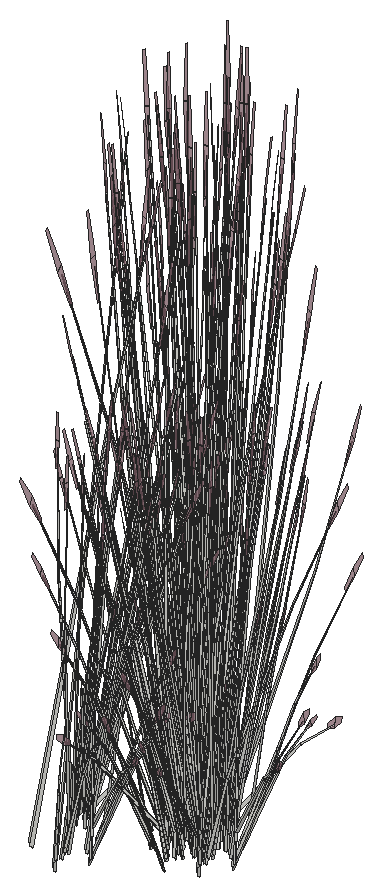
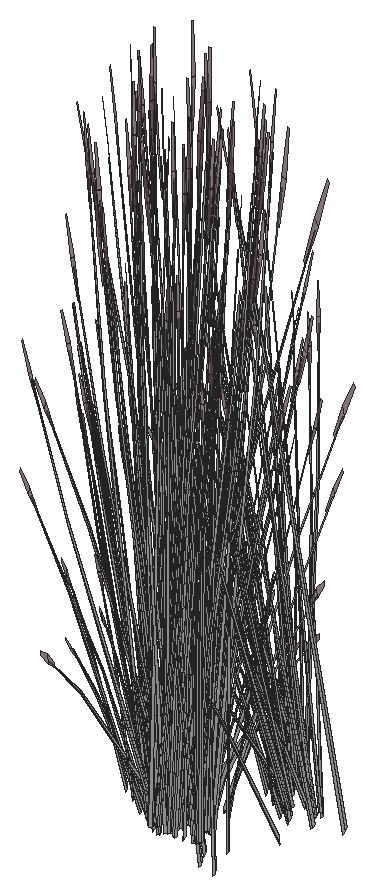
# SketchUp Ruby script. Lengths in inches.
U = 1.inch
M = Sketchup.active_model
def pt(a) = Geom::Point3d.new(a.map { |v| v * U })
def face(e, loops, mat)
  f = e.add_face(loops[0].map { |a| pt(a) })
  loops[1..].each { |l| e.add_face(l.map { |a| pt(a) }).erase! }
  f.material = f.back_material = mat if mat
  f
end
# faces: each face lists its corners as indices into pts; further lists are holes
def faces(e, pts, list, mat = nil) = list.each { |f| face(e, (f[0].is_a?(Array) ? f : [f]).map { |l| l.map { |i| pts[i] } }, mat) }
# xy, xz, yz: faces in a plane at the given z, y or x. An outline is a flat list of corners, or four numbers for a rectangle; further outlines are holes
def ring(l) = l.size == 4 ? [[l[0], l[1]], [l[2], l[1]], [l[2], l[3]], [l[0], l[3]]] : l.each_slice(2).to_a
def flat(e, list, mat, &to3) = list.each { |f| face(e, (f[0].is_a?(Array) ? f : [f]).map { |l| ring(l).map { |u, v| to3.(u, v) } }, mat) }
def xy(e, z, list, mat = nil) = flat(e, list, mat) { |x, y| [x, y, z] }
def xz(e, y, list, mat = nil) = flat(e, list, mat) { |x, z| [x, y, z] }
def yz(e, x, list, mat = nil) = flat(e, list, mat) { |y, z| [x, y, z] }
def lines(e, pts, list) = list.each { |a, b| e.add_line(pt(pts[a]), pt(pts[b])) }
# prism: a flat outline (further loops are holes) pulled along v
def prism(e, loops, v, mat = nil)
  f = face(e, loops, mat); d = Geom::Vector3d.new(v.map { |x| x * U })
  f.pushpull(f.normal.samedirection?(d) ? d.length : -d.length)
end
def box(e, o, s, mat = nil) = prism(e, [[o, [o[0] + s[0], o[1], o[2]], [o[0] + s[0], o[1] + s[1], o[2]], [o[0], o[1] + s[1], o[2]]]], [0, 0, s[2]], mat)
def at(x, y, z, deg = 0) = Geom::Transformation.translation(pt([x, y, z])) * Geom::Transformation.rotation(ORIGIN, Z_AXIS, deg.degrees)
def axes(o, x, y, z) = Geom::Transformation.new([*x, 0, *y, 0, *z, 0, *pt(o).to_a, 1])
def part(name) = M.definitions.add(name)
# library, detail: a bought-in or finely detailed component or shape, given as its bounding box
def library(name, o, s) = part(name).tap { |d| box(d.entities, o, s) }
def detail(e, o, s) = box(e.add_group.entities, o, s)
def put(e, d, t, mat = nil) = e.add_instance(d, t).tap { |i| i.material = mat if mat }
def group(e, t, mat = nil) = e.add_group.tap { |g| g.transformation = t; g.material = mat if mat }.entities
root = M.entities
M.materials.add("LightPink_Translucent").color = [144, 107, 117]
M.materials["LightPink_Translucent"].alpha = 0.75
c1 = part("blade")
p = [[2.15,0.21,22],[0,0.17,0],[0.09,0.45,0],[2.18,0.31,22],[2.29,0.31,22],[0.38,0.45,0],
  [2.48,0.24,33],[2.49,0.24,33],[2.48,0.22,33]]
faces(c1.entities,p,[[0,1,2,3],[4,5,2,3],[6,3,4,7],[8,0,3,6]])
c2 = part("seeds")
p = [[0.3,-0.1,1.38],[-0.01,-0.03,1.59],[-0.01,-0.03,0.03],[0.14,-0.07,-0.07],[0.29,-0.03,3],[0.15,0.01,3.11]]
faces(c2.entities,p,[[0,1,2,3],[1,0,4,5]],"LightPink_Translucent")
c3 = part("blade with seeds")
put(c3.entities,c1,at(0,0,0))
put(c3.entities,c2,axes([2.4,0.25,30.99],[1.5799,-0.05474,1.17369],[-0.12525,1.92788,0.29478],[-0.07173,-0.02425,1.56792]))
put(root,c3,axes([405.3125,10.01,-10.61],[-0.07655,-0.04282,1.6421],[-0.19662,-0.47839,-0.25086],[0.13264,-0.12982,0.2797]))
put(root,c3,axes([405.3125,11.36,-7.36],[0.26714,-0.42887,-0.66157],[0.46811,0.30479,0.07984],[0.1595,-0.15539,0.93586]))
put(root,c3,axes([405.3,11.16,-7.64],[-0.13138,-0.49631,-0.47583],[0.49754,-0.08682,-0.36857],[0.14258,-0.13331,0.91046]))
put(root,c3,axes([405.53,11.52,-7.3125],[-0.47307,-0.29971,-0.11324],[0.27254,-0.43404,-0.62851],[0.13365,-0.15087,0.95501]))
put(root,c3,axes([405.7,10.97,-9.59],[-0.1827,-0.0161,1.33163],[-0.18717,-0.43188,-0.28638],[0.22444,-0.12218,0.56934]))
put(root,c3,axes([406.7,11.39,-7.62],[-0.0668,-0.00413,1.65179],[-0.27738,-0.44233,-0.15608],[0.11139,-0.14544,0.29231]))
put(root,c3,axes([405.91,10.18,-9.42],[-0.17034,0.27669,1.06958],[-0.14642,-0.37174,0.78586],[0.14069,-0.09315,0.23558]))
put(root,c3,axes([405.66,11.22,-7.78],[0.44516,-0.07768,-0.32977],[0.11755,0.44407,0.42575],[0.12757,-0.11927,0.81462]))
put(root,c3,axes([405.7,11.41,-7.6],[0.35109,0.22859,0.05988],[-0.2044,0.32553,0.47138],[0.11256,-0.10524,0.71878]))
put(root,c3,axes([405.61,11.3125,-7.59],[0.12683,0.50025,0.447],[-0.49754,0.08682,0.36857],[0.14663,-0.11765,0.92496]))
put(root,c3,axes([406.95,11.92,-7.61],[0.07097,-0.08279,1.62908],[-0.09083,-0.50786,-0.25764],[0.17806,-0.09629,0.13065]))
put(root,c3,axes([409.84,15.22,-8.39],[0.1169,0.17452,1.59586],[-0.54019,0.14692,0.12904],[-0.12209,-0.27397,0.68222]))
put(root,c3,axes([410.73,14.06,-7.61],[-0.07822,-0.07621,1.62908],[-0.52201,0.04832,-0.25764],[-0.08331,-0.18228,0.13065]))
put(root,c3,axes([411.94,14.97,-9.59],[-0.14537,0.11002,1.33163],[-0.43536,-0.19256,-0.28638],[0.0807,-0.23948,0.56934]))
put(root,c3,axes([405.55,12.6875,-7.3125],[-0.25732,-0.49218,-0.11324],[0.45669,-0.24187,-0.62851],[0.19245,-0.06494,0.95501]))
put(root,c3,axes([405.53,12.27,-7.64],[0.13855,-0.49442,-0.47583],[0.47502,0.16947,-0.36857],[0.19125,-0.04534,0.91046]))
put(root,c3,axes([404.78,10.25,-9.79],[0.31974,-0.54466,0],[0.53494,0.30375,-0.48057],[0.12184,0.06918,1.52448]))
put(root,c3,axes([411.28,15.35,-7.36],[-0.24409,-0.44196,-0.66157],[0.50245,-0.2463,0.07984],[-0.05708,-0.21354,0.93586]))
put(root,c3,axes([409.69,14.76,-9.59],[-0.03097,0.17781,1.33163],[-0.45273,0.14885,-0.28638],[-0.10583,-0.22982,0.56934]))
put(root,c3,axes([406.04,12.4,-10.15],[-0.32938,0.06523,1.31842],[-0.05243,-0.51922,0.07547],[0.2307,-0.07859,0.75023]))
put(root,c3,axes([406.64,11.94,-9.89],[-0.31706,-0.34757,-0.06041],[0.34725,-0.31847,-0.27392],[0.09839,-0.02242,0.90349]))
put(root,c3,axes([410.86,14.37,-10.61],[-0.08578,0.01958,1.6421],[-0.47437,-0.22044,-0.25086],[0.00796,-0.18387,0.2797]))
put(root,c3,axes([405.4375,12.45,-7.36],[0.44939,-0.24006,-0.66157],[0.25044,0.49415,0.07984],[0.21713,-0.05613,0.93586]))
put(root,c3,axes([412.29,15.78,-7.36],[0.01331,-0.50278,-0.66157],[0.56035,0.03377,0.07984],[0.05914,-0.213,0.93586]))
put(root,c3,axes([413.08,15,-7.61],[-0.00494,-0.10818,1.62908],[-0.41695,-0.31265,-0.25764],[0.06446,-0.18952,0.13065]))
put(root,c3,axes([411.32,14.98,-7.78],[0.15418,-0.41799,-0.32977],[0.44981,0.12192,0.42575],[-0.04124,-0.16829,0.81462]))
put(root,c3,axes([411.66,15.53,-8.39],[-0.09522,0.18683,1.59586],[-0.39947,-0.38663,0.12904],[0.18021,-0.24097,0.68222]))
put(root,c3,axes([412.96,14.61,-7.62],[-0.05194,0.04152,1.65179],[-0.50886,-0.14007,-0.15608],[-0.01842,-0.18118,0.29231]))
put(root,c3,axes([405.37,12.54,-7.3],[-0.42502,-0.15163,0.32977],[0.12396,-0.44238,-0.42575],[0.17112,-0.04056,0.81462]))
put(root,c3,axes([411.1,15.26,-7.64],[-0.50273,-0.13626,-0.47583],[0.17232,-0.46717,-0.36857],[-0.0461,-0.18809,0.91046]))
put(root,c3,axes([411.41,14.09,-9.42],[0.06561,0.31695,1.06958],[-0.36394,-0.17555,0.78586],[0.03916,-0.16229,0.23558]))
put(root,c3,axes([402.46,11.22,-10.52],[-0.50338,0.21762,1.20058],[-0.16022,-0.62439,0.4665],[0.30911,0.01039,1.36553]))
put(root,c3,axes([412.18,15.62,-7.64],[-0.3661,-0.36521,-0.47583],[0.38674,-0.31985,-0.36857],[0.0557,-0.18556,0.91046]))
put(root,c3,axes([406.4,12.07,-10.61],[-0.02673,-0.08252,1.6421],[0.18538,-0.48271,-0.25086],[0.187,-0.00694,0.2797]))
put(root,c3,axes([410.2,13.82,-7.62],[-0.00954,0.06515,1.65179],[-0.47055,0.23645,-0.15608],[-0.13847,-0.12087,0.29231]))
put(root,c3,axes([410.09,14.97,-7.26],[0.56969,-0.13971,0.50064],[0.09887,0.54803,0.4128],[-0.13398,-0.16152,1.03595]))
put(root,c3,axes([411.38,15.07,-7.59],[0.50393,0.1421,0.447],[-0.17232,0.46717,0.36857],[-0.03028,-0.18372,0.92496]))
put(root,c3,axes([405.82,12.49,-7.78],[0.42502,0.15163,-0.32977],[-0.12396,0.44238,0.42575],[0.17112,-0.04056,0.81462]))
put(root,c3,axes([411.53,15.24,-7.3125],[-0.50045,0.25306,-0.11324],[-0.24593,-0.44915,-0.62851],[-0.06603,-0.18927,0.95501]))
put(root,c3,axes([412.57,15.81,-7.3125],[-0.56206,-0.02693,-0.11324],[0.01536,-0.50991,-0.62851],[0.03904,-0.19638,0.95501]))
put(root,c3,axes([412.53,15.48,-7.78],[0.34603,-0.28618,-0.32977],[0.32756,0.32677,0.42575],[0.04984,-0.16603,0.81462]))
put(root,c3,axes([409.54,14.47,-9.42],[0.26677,0.18918,1.06958],[-0.38851,0.11372,0.78586],[-0.08313,-0.14539,0.23558]))
put(root,c3,axes([411.51,15.04,-7.6],[0.37684,-0.18473,0.05988],[0.18445,0.33686,0.47138],[-0.03639,-0.14849,0.71878]))
put(root,c3,axes([405.07,10.58,-10.12],[0.47863,0.27177,-0.46235],[-0.28609,0.48733,0],[0.10901,0.0619,1.46668]))
put(root,c3,axes([410.03,15.13,-7.78],[-0.07899,-0.43781,-0.32977],[0.45153,-0.11561,0.42575],[-0.12128,-0.12546,0.81462]))
put(root,c3,axes([404.66,11.94,-8.39],[-0.21212,0.01231,1.59586],[0.14072,-0.53355,0.12904],[0.3023,0.033,0.68222]))
put(root,c3,axes([405.76,12.68,-7.6],[0.18783,0.37061,0.05988],[-0.34252,0.1814,0.47138],[0.15099,-0.03579,0.71878]))
put(root,c3,axes([410.22,15.09,-7.6],[0.23243,-0.34529,0.05988],[0.331,0.20103,0.47138],[-0.10701,-0.1107,0.71878]))
put(root,c3,axes([405.72,12.55,-7.59],[-0.14449,0.4956,0.447],[-0.47502,-0.16947,0.36857],[0.1868,-0.02978,0.92496]))
put(root,c3,axes([410.15,17.01,-10.05],[-0.21003,-0.55738,-0.65031],[0.60499,-0.20074,-0.17068],[-0.02321,-0.18874,1.43544]))
put(root,c3,axes([412.96,15.31,-10.61],[-0.07655,-0.04282,1.6421],[-0.19662,-0.47839,-0.25086],[0.13264,-0.12982,0.2797]))
put(root,c3,axes([411.375,15.42,-7.3],[-0.15418,0.41799,0.32977],[-0.44981,-0.12192,-0.42575],[-0.04124,-0.16829,0.81462]))
put(root,c3,axes([412.52,15.59,-7.59],[0.36417,0.37086,0.447],[-0.38674,0.31985,0.36857],[0.06718,-0.174,0.92496]))
put(root,c3,axes([404.37,11.62,-10.08],[0.53199,0.08911,-0.58063],[-0.11226,0.54969,-0.15239],[0.15876,0.06661,1.28164]))
put(root,c3,axes([412.66,15.63,-7.6],[0.42027,0.02533,0.05988],[-0.01152,0.38243,0.47138],[0.04398,-0.14649,0.71878]))
put(root,c3,axes([406.72,12.58,-9.42],[-0.31598,0.08973,1.06958],[0.14873,-0.37085,0.78586],[0.16763,0.02538,0.23558]))
put(root,c3,axes([412.34,15.89,-7.3],[-0.34603,0.28618,0.32977],[-0.32756,-0.32677,-0.42575],[0.04984,-0.16603,0.81462]))
put(root,c3,axes([412.96,16.66,-7.36],[0.26714,-0.42887,-0.66157],[0.46811,0.30479,0.07984],[0.1595,-0.15539,0.93586]))
put(root,c3,axes([410.07,15.41,-9.79],[-0.31974,-0.54466,0],[0.53494,-0.30375,-0.48057],[0.12184,-0.06918,1.52448]))
put(root,c3,axes([412.94,16.46,-7.64],[-0.13138,-0.49631,-0.47583],[0.49754,-0.08682,-0.36857],[0.14258,-0.13331,0.91046]))
put(root,c3,axes([410.77,14.75,-10.02],[-0.35341,0.31182,-0.03625],[-0.32382,-0.34152,-0.16435],[-0.0228,-0.09677,0.54209]))
put(root,c3,axes([406.57,14.15,-7.62],[-0.04624,-0.04758,1.65179],[0.10116,-0.51007,-0.15608],[0.18215,-0.03259,0.29231]))
put(root,c3,axes([413.18,16.8125,-7.3125],[-0.47307,-0.29971,-0.11324],[0.27254,-0.43404,-0.62851],[0.13365,-0.15087,0.95501]))
put(root,c3,axes([406.17,13.72,-8.34],[-0.09788,-0.45691,-0.03251],[0.46264,-0.10504,-0.14742],[0.09661,0.02897,0.48626]))
put(root,c3,axes([404.97,13.71,-7.3125],[0.02738,-0.55277,-0.11324],[0.51847,0.01511,-0.62851],[0.19968,0.0384,0.95501]))
put(root,c3,axes([411.22,18.45,-8.9],[0.44194,0.21918,1.40854],[-0.43295,0.47219,0.557],[-0.19393,-0.27986,1.18082]))
put(root,c3,axes([404.89,13.49,-7.3],[-0.29098,-0.34031,0.32977],[0.33226,-0.32215,-0.42575],[0.16881,0.04902,0.81462]))
put(root,c3,axes([410.29,15.49,-7.3],[0.07899,0.43781,0.32977],[-0.45153,0.11561,-0.42575],[-0.12128,-0.12546,0.81462]))
put(root,c3,axes([408.91,16.93,-10.12],[0,-0.54355,-0.46235],[0.57217,0,0],[0,-0.1238,1.46668]))
put(root,c3,axes([410.5,15.33,-10.12],[0.47863,-0.27177,-0.46235],[0.28609,0.48733,0],[0.10901,-0.0619,1.46668]))
put(root,c3,axes([413.34,16.26,-9.59],[-0.1827,-0.0161,1.33163],[-0.18717,-0.43188,-0.28638],[0.22444,-0.12218,0.56934]))
put(root,c3,axes([414.34,16.68,-7.62],[-0.0668,-0.00413,1.65179],[-0.27738,-0.44233,-0.15608],[0.11139,-0.14544,0.29231]))
put(root,c3,axes([406.13,13.18,-9.59],[-0.12317,-0.13368,1.33163],[0.16025,-0.44223,-0.28638],[0.24919,0.05991,0.56934]))
put(root,c3,axes([411.07,16.44,-10.08],[0.34446,-0.40855,-0.58063],[0.42791,0.37046,-0.15239],[0.13803,-0.10191,1.28164]))
put(root,c3,axes([413.55,15.47,-9.42],[-0.17034,0.27669,1.06958],[-0.14642,-0.37174,0.78586],[0.14069,-0.09315,0.23558]))
put(root,c3,axes([405.42,13.38,-7.61],[0.10971,-0.00919,1.62908],[0.30091,-0.42228,-0.25764],[0.19514,0.05574,0.13065]))
put(root,c3,axes([413.31,16.51,-7.78],[0.44516,-0.07768,-0.32977],[0.11755,0.44407,0.42575],[0.12757,-0.11927,0.81462]))
put(root,c3,axes([410.47,17.16,-9.94],[0.24813,-0.48978,-0.41661],[0.51557,0.23571,0.2005],[0,-0.1129,1.33761]))
put(root,c3,axes([410.7,16.91,-9.52],[-0.05959,-0.62022,-0.27094],[0.62068,-0.0375,-0.46562],[0.1093,-0.08261,1.4872]))
put(root,c3,axes([409.16,16.95,-10.11],[0.35699,-0.33913,-0.28847],[0.35699,0.33913,0.28847],[0,-0.10923,1.29413]))
put(root,c3,axes([409.01,15.32,-10.02],[-0.14753,0.44383,-0.03625],[-0.45406,-0.13653,-0.16435],[-0.06894,-0.07259,0.54209]))
put(root,c3,axes([405,13.45,-7.36],[0.51122,0.01309,-0.66157],[-0.03434,0.5511,0.07984],[0.21658,0.05816,0.93586]))
put(root,c3,axes([412.95,16.77,-7.3],[-0.44516,0.07768,0.32977],[-0.11755,-0.44407,-0.42575],[0.12757,-0.11927,0.81462]))
put(root,c3,axes([410.41,17.5625,-9.52],[-0.57594,-0.25935,-0.27094],[0.27732,-0.5474,-0.46562],[-0.0181,-0.1344,1.4872]))
put(root,c3,axes([408.77,17.35,-9.79],[-0.63949,0,0],[0,-0.60749,-0.48057],[0,-0.13836,1.52448]))
put(root,c3,axes([410.61,15.54,-10.11],[0.47712,0.13449,-0.28847],[-0.12013,0.47362,0.28847],[0.09619,-0.05462,1.29413]))
put(root,c3,axes([405.31,13.67,-7.78],[0.29098,0.34031,-0.32977],[-0.33226,0.32215,0.42575],[0.16881,0.04902,0.81462]))
put(root,c3,axes([405.16,13.8,-7.6],[-0.02575,0.41332,0.05988],[-0.38885,-0.01133,0.47138],[0.14895,0.04325,0.71878]))
put(root,c3,axes([413.35,16.7,-7.6],[0.35109,0.22859,0.05988],[-0.2044,0.32553,0.47138],[0.11256,-0.10524,0.71878]))
put(root,c3,axes([413.25,16.61,-7.59],[0.12683,0.50025,0.447],[-0.49754,0.08682,0.36857],[0.14663,-0.11765,0.92496]))
put(root,c3,axes([414.59,17.21,-7.61],[0.07097,-0.08279,1.62908],[-0.09083,-0.50786,-0.25764],[0.17806,-0.09629,0.13065]))
put(root,c3,axes([405.19,13.67,-7.59],[-0.37709,0.35815,0.447],[-0.32522,-0.38035,0.36857],[0.17692,0.06607,0.92496]))
put(root,c3,axes([409.26,17.1875,-9.83],[-0.47569,0.45698,0.2864],[-0.47598,-0.45217,-0.33981],[-0.01661,-0.12977,1.53541]))
put(root,c3,axes([410.78,17.4,-9.73],[0.57623,0.26344,0.22409],[-0.27732,0.5474,0.46562],[0,-0.12618,1.49497]))
put(root,c3,axes([410.55,18.14,-9.73],[0.13555,-0.64407,-0.21817],[0.64269,0.11227,0.47743],[-0.1123,-0.08895,1.45677]))
put(root,c3,axes([404.26,12.8,-8.39],[-0.18996,-0.09365,1.59586],[0.39312,-0.39287,0.12904],[0.24502,0.17723,0.68222]))
put(root,c3,axes([410.59,17.03,-9.47],[-0.55535,0.03355,0.41661],[-0.05022,-0.55698,-0.2005],[0.09942,-0.05645,1.33761]))
put(root,c3,axes([409.16,17.4375,-9.69],[0,0.54355,0.46235],[-0.57217,0,0],[0,-0.1238,1.46668]))
put(root,c3,axes([413.2,17.98,-7.3125],[-0.25732,-0.49218,-0.11324],[0.45669,-0.24187,-0.62851],[0.19245,-0.06494,0.95501]))
put(root,c3,axes([413.17,17.56,-7.64],[0.13855,-0.49442,-0.47583],[0.47502,0.16947,-0.36857],[0.19125,-0.04534,0.91046]))
put(root,c3,axes([403.95,14.3125,-7.3125],[0.30474,-0.46525,-0.11324],[0.44133,0.26804,-0.62851],[0.15341,0.13145,0.95501]))
put(root,c3,axes([412.42,15.55,-9.79],[0.31974,-0.54466,0],[0.53494,0.30375,-0.48057],[0.12184,0.06918,1.52448]))
put(root,c3,axes([410.51,17.88,-9.94],[-0.30722,-0.45622,-0.41661],[0.46535,-0.32126,0.2005],[-0.09942,-0.05645,1.33761]))
put(root,c3,axes([410.57,17.23,-9.8],[0.22235,0.6078,0.42607],[-0.63531,0.21135,0.16719],[0.00776,-0.11168,1.47927]))
put(root,c3,axes([413.68,17.7,-10.15],[-0.32938,0.06523,1.31842],[-0.05243,-0.51922,0.07547],[0.2307,-0.07859,0.75023]))
put(root,c3,axes([414.28,17.24,-9.89],[-0.31706,-0.34757,-0.06041],[0.34725,-0.31847,-0.27392],[0.09839,-0.02242,0.90349]))
put(root,c3,axes([410.46,17.71,-9.47],[-0.24813,0.48978,0.41661],[-0.51557,-0.23571,-0.2005],[0,-0.1129,1.33761]))
put(root,c3,axes([411.37,17.28,-9.95],[0,-0.62892,0],[0.63949,0,0],[0,0,1.6711]))
put(root,c3,axes([405.04,14.45,-10.61],[0.03726,-0.07847,1.6421],[0.46909,-0.23111,-0.25086],[0.14221,0.11962,0.2797]))
put(root,c3,axes([412.15,15.83,-9.69],[-0.47863,-0.27177,0.46235],[0.28609,-0.48733,0],[0.10901,0.0619,1.46668]))
put(root,c3,axes([413.08,17.74,-7.36],[0.44939,-0.24006,-0.66157],[0.25044,0.49415,0.07984],[0.21713,-0.05613,0.93586]))
put(root,c3,axes([404.3125,14.08,-7.64],[0.50465,-0.12921,-0.47583],[0.08828,0.48932,-0.36857],[0.13555,0.14022,0.91046]))
put(root,c3,axes([411.07,16.89,-9.8],[-0.42403,0.49328,0.42607],[-0.50377,-0.43543,0.16719],[0.10223,-0.04923,1.47927]))
put(root,c3,axes([404.64,20.83,-8.39],[-0.09522,0.18683,1.59586],[-0.39947,-0.38663,0.12904],[0.18021,-0.24097,0.68222]))
put(root,c3,axes([411.53,17.77,-9.86],[-0.47569,-0.46784,-0.05709],[0.47598,-0.46812,0],[-0.01661,-0.01634,1.63492]))
put(root,c3,axes([410.33,16.08,-9.7],[-0.14774,0.54019,0.16428],[-0.54062,-0.15287,0.32672],[0.09339,-0.00263,1.49371]))
put(root,c3,axes([413.02,17.83,-7.3],[-0.42502,-0.15163,0.32977],[0.12396,-0.44238,-0.42575],[0.17112,-0.04056,0.81462]))
put(root,c3,axes([410.11,16.51,-10.52],[-0.50338,0.21762,1.20058],[-0.16022,-0.62439,0.4665],[0.30911,0.01039,1.36553]))
put(root,c3,axes([411.46,16.68,-9.5625],[0.09866,-0.48509,0.13483],[0.48202,0.0842,-0.38503],[0.08772,0.04981,1.18024]))
put(root,c3,axes([410.625,17.83,-9.8],[0.64638,0.11452,0.42607],[-0.13155,0.64678,0.16719],[-0.09446,-0.06245,1.47927]))
put(root,c3,axes([414.04,17.36,-10.61],[-0.02673,-0.08252,1.6421],[0.18538,-0.48271,-0.25086],[0.187,-0.00694,0.2797]))
put(root,c3,axes([411.25,16.8,-9.47],[-0.30722,-0.45622,0.41661],[0.46535,-0.32126,-0.2005],[0.09942,0.05645,1.33761]))
put(root,c3,axes([409.67,18.89,-10.11],[-0.12013,-0.47362,-0.28847],[0.47712,-0.13449,0.28847],[-0.09619,-0.05462,1.29413]))
put(root,c3,axes([410.28,18.86,-9.7],[0.54955,-0.14427,0.16428],[0.1357,0.53689,0.32672],[-0.04901,-0.07823,1.49371]))
put(root,c3,axes([411.41,16.83,-9.52],[0.51635,-0.36087,-0.27094],[0.34336,0.5099,-0.46562],[0.1274,0.05178,1.4872]))
put(root,c3,axes([413.46,17.79,-7.78],[0.42502,0.15163,-0.32977],[-0.12396,0.44238,0.42575],[0.17112,-0.04056,0.81462]))
put(root,c3,axes([412.71,15.875,-10.12],[0.47863,0.27177,-0.46235],[-0.28609,0.48733,0],[0.10901,0.0619,1.46668]))
put(root,c3,axes([411.8,17.43,-9.95],[0.57217,0,0],[0,0.56272,0],[0,0,1.66132]))
put(root,c3,axes([410.84,18.13,-9.52],[-0.51635,0.36087,-0.27094],[-0.34336,-0.5099,-0.46562],[-0.1274,-0.05178,1.4872]))
put(root,c3,axes([411.97,16.11,-9.7],[-0.54955,0.14427,0.16428],[-0.1357,-0.53689,0.32672],[0.04901,0.07823,1.49371]))
put(root,c3,axes([412.31,17.24,-8.39],[-0.21212,0.01231,1.59586],[0.14072,-0.53355,0.12904],[0.3023,0.033,0.68222]))
put(root,c3,axes([412.58,16.08,-10.11],[0.12013,0.47362,-0.28847],[-0.47712,0.13449,0.28847],[0.09619,0.05462,1.29413]))
put(root,c3,axes([413.4,17.97,-7.6],[0.18783,0.37061,0.05988],[-0.34252,0.1814,0.47138],[0.15099,-0.03579,0.71878]))
put(root,c3,axes([411.62,17.14,-9.78],[-0.64638,-0.11452,0.45814],[0.13155,-0.64678,0.17978],[0.09446,0.06245,1.59061]))
put(root,c3,axes([413.37,17.84,-7.59],[-0.14449,0.4956,0.447],[-0.47502,-0.16947,0.36857],[0.1868,-0.02978,0.92496]))
put(root,c3,axes([411.1,18.74,-9.95],[-0.16686,-0.46861,0],[0.47648,-0.16411,0],[0,0,1.4375]))
put(root,c3,axes([410.79,18.29,-9.5625],[-0.09866,0.48509,0.13483],[-0.48202,-0.0842,-0.38503],[-0.08772,-0.04981,1.18024]))
put(root,c3,axes([405.93,20.61,-10.61],[-0.07655,-0.04282,1.6421],[-0.19662,-0.47839,-0.25086],[0.13264,-0.12982,0.2797]))
put(root,c3,axes([411.73,18.67,-9.97],[0.53691,-0.18442,-0.17877],[0.18866,0.53125,0.00007],[0.05927,-0.02038,1.61933]))
put(root,c3,axes([411.92,18.89,-9.7],[0.14774,-0.54019,0.16428],[0.54062,0.15287,0.32672],[-0.09339,0.00263,1.49371]))
put(root,c3,axes([411.79,17.67,-9.9375],[0.35699,0.35109,0],[-0.35699,0.35109,0],[0,0,1.57621]))
put(root,c3,axes([412.76,17.51,-9.7],[-0.40181,-0.39593,0.16428],[0.40492,-0.38402,0.32672],[-0.04438,0.08086,1.49371]))
put(root,c3,axes([412.02,16.92,-10.08],[0.53199,0.08911,-0.58063],[-0.11226,0.54969,-0.15239],[0.15876,0.06661,1.28164]))
put(root,c3,axes([414.37,17.875,-9.42],[-0.31598,0.08973,1.06958],[0.14873,-0.37085,0.78586],[0.16763,0.02538,0.23558]))
put(root,c3,axes([410.99,18.95,-9.95],[-0.51557,-0.24403,0],[0.24813,-0.50705,0],[0,0,1.51513]))
put(root,c3,axes([411.42,18.3,-9.7],[-0.49938,-0.43748,-0.23459],[0.42021,-0.49126,0.51337],[-0.13447,0.05118,1.56642]))
put(root,c3,axes([410.1,19.14,-9.69],[0.47863,0.27177,0.46235],[-0.28609,0.48733,0],[-0.10901,-0.0619,1.46668]))
put(root,c3,axes([405.93,21.96,-7.36],[0.26714,-0.42887,-0.66157],[0.46811,0.30479,0.07984],[0.1595,-0.15539,0.93586]))
put(root,c3,axes([405.92,21.76,-7.64],[-0.13138,-0.49631,-0.47583],[0.49754,-0.08682,-0.36857],[0.14258,-0.13331,0.91046]))
put(root,c3,axes([411.79,17.26,-9.47],[0.24813,-0.48978,0.41661],[0.51557,0.23571,-0.2005],[0,0.1129,1.33761]))
put(root,c3,axes([414.22,19.44,-7.62],[-0.04624,-0.04758,1.65179],[0.10116,-0.51007,-0.15608],[0.18215,-0.03259,0.29231]))
put(root,c3,axes([411.69,17.54,-9.87],[0,0.62861,-0.05249],[-0.63949,0,0],[0,0.01975,1.67027]))
put(root,c3,axes([411.74,17.09,-9.94],[0.30722,0.45622,-0.41661],[-0.46535,0.32126,0.2005],[0.09942,0.05645,1.33761]))
put(root,c3,axes([413.82,19.02,-8.34],[-0.09788,-0.45691,-0.03251],[0.46264,-0.10504,-0.14742],[0.09661,0.02897,0.48626]))
put(root,c3,axes([406.15,22.12,-7.3125],[-0.47307,-0.29971,-0.11324],[0.27254,-0.43404,-0.62851],[0.13365,-0.15087,0.95501]))
put(root,c3,axes([412.62,19.01,-7.3125],[0.02738,-0.55277,-0.11324],[0.51847,0.01511,-0.62851],[0.19968,0.0384,0.95501]))
put(root,c3,axes([413.09,17.53,-9.69],[0,-0.54355,0.46235],[0.57217,0,0],[0,0.1238,1.46668]))
put(root,c3,axes([411.66,17.94,-9.47],[0.55535,-0.03355,0.41661],[0.05022,0.55698,-0.2005],[-0.09942,0.05645,1.33761]))
put(root,c3,axes([412,17.37,-9.5625],[0.47648,-0.15851,0.13483],[0.16686,0.45265,-0.38503],[0,0.09962,1.18024]))
put(root,c3,axes([412.54,18.79,-7.3],[-0.29098,-0.34031,0.32977],[0.33226,-0.32215,-0.42575],[0.16881,0.04902,0.81462]))
put(root,c3,axes([411.16,18.21,-9.94],[-0.55535,0.03355,-0.41661],[-0.05022,-0.55698,0.2005],[-0.09942,0.05645,1.33761]))
put(root,c3,axes([406.32,21.57,-9.59],[-0.1827,-0.0161,1.33163],[-0.18717,-0.43188,-0.28638],[0.22444,-0.12218,0.56934]))
put(root,c3,axes([407.32,21.99,-7.62],[-0.0668,-0.00413,1.65179],[-0.27738,-0.44233,-0.15608],[0.11139,-0.14544,0.29231]))
put(root,c3,axes([413.77,18.47,-9.59],[-0.12317,-0.13368,1.33163],[0.16025,-0.44223,-0.28638],[0.24919,0.05991,0.56934]))
put(root,c3,axes([406.53,20.77,-9.42],[-0.17034,0.27669,1.06958],[-0.14642,-0.37174,0.78586],[0.14069,-0.09315,0.23558]))
put(root,c3,axes([411.57,18.96,-9.95],[0.51557,0.24403,0],[-0.24813,0.50705,0],[0,0,1.62917]))
put(root,c3,axes([413.07,18.67,-7.61],[0.10971,-0.00919,1.62908],[0.30091,-0.42228,-0.25764],[0.19514,0.05574,0.13065]))
put(root,c3,axes([411.78,19.5,-9.96],[-0.31576,-0.54657,-0.04789],[0.53494,-0.30375,0.48057],[-0.13182,0.05204,1.52373]))
put(root,c3,axes([411.67,18.17,-9.5625],[0.37783,0.32657,0.13483],[-0.31516,0.36844,-0.38503],[-0.08772,0.04981,1.18024]))
put(root,c3,axes([406.28,21.8125,-7.78],[0.44516,-0.07768,-0.32977],[0.11755,0.44407,0.42575],[0.12757,-0.11927,0.81462]))
put(root,c3,axes([412.64,18.74,-7.36],[0.51122,0.01309,-0.66157],[-0.03434,0.5511,0.07984],[0.21658,0.05816,0.93586]))
put(root,c3,axes([405.92,22.08,-7.3],[-0.44516,0.07768,0.32977],[-0.11755,-0.44407,-0.42575],[0.12757,-0.11927,0.81462]))
put(root,c3,axes([412.07,19.18,-9.69],[0.47863,-0.27177,0.46235],[0.28609,0.48733,0],[-0.10901,0.0619,1.46668]))
put(root,c3,axes([411.39,18.75,-9.87],[0.22235,0.62444,-0.05599],[-0.63531,0.21881,0],[0.00776,0.02181,1.60327]))
put(root,c3,axes([411.63,19.43,-10.11],[-0.47712,-0.13449,-0.28847],[0.12013,-0.47362,0.28847],[-0.09619,0.05462,1.29413]))
put(root,c3,axes([408.99,18.09,-7.3],[0.44516,-0.07768,0.32977],[0.11755,0.44407,-0.42575],[-0.12757,0.11927,0.81462]))
put(root,c3,axes([413.48,17.62,-9.79],[0.63949,0,0],[0,0.60749,-0.48057],[0,0.13836,1.52448]))
put(root,c3,axes([413.22,17.93,-9.95],[-0.63917,-0.00435,-0.04634],[0,-0.60749,0.46507],[-0.02009,0.13829,1.47457]))
put(root,c3,axes([411.84,17.4,-9.52],[0.57594,0.25935,-0.27094],[-0.27732,0.5474,-0.46562],[0.0181,0.1344,1.4872]))
